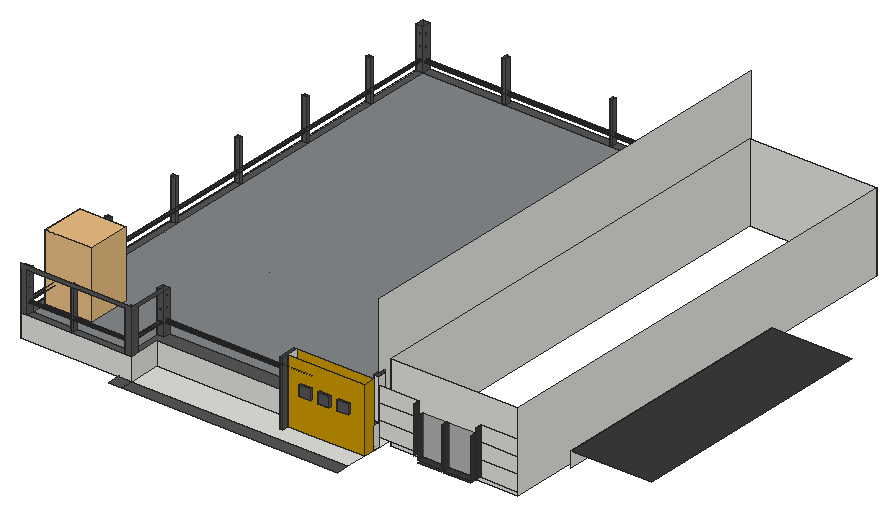
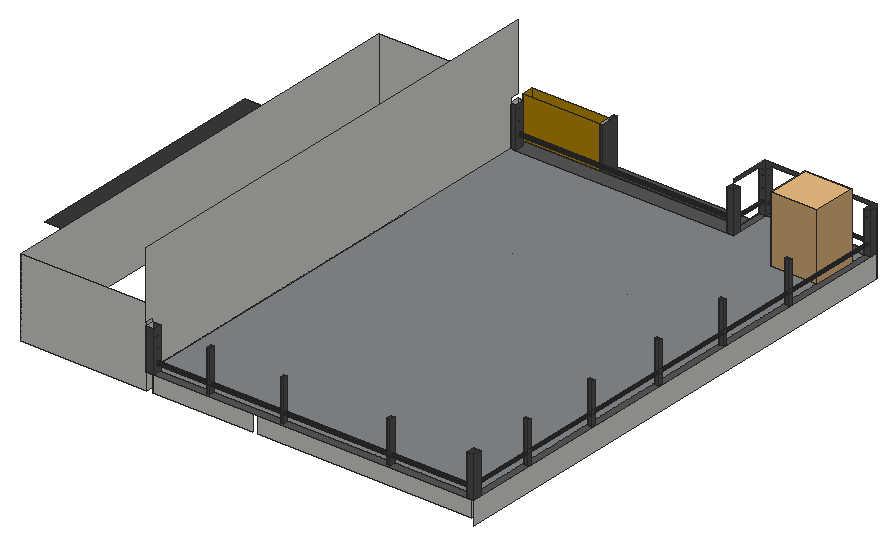
# SketchUp Ruby script. Lengths in inches.
U = 1.inch
M = Sketchup.active_model
def pt(a) = Geom::Point3d.new(a.map { |v| v * U })
def face(e, loops, mat)
  f = e.add_face(loops[0].map { |a| pt(a) })
  loops[1..].each { |l| e.add_face(l.map { |a| pt(a) }).erase! }
  f.material = f.back_material = mat if mat
  f
end
# faces: each face lists its corners as indices into pts; further lists are holes
def faces(e, pts, list, mat = nil) = list.each { |f| face(e, (f[0].is_a?(Array) ? f : [f]).map { |l| l.map { |i| pts[i] } }, mat) }
# xy, xz, yz: faces in a plane at the given z, y or x. An outline is a flat list of corners, or four numbers for a rectangle; further outlines are holes
def ring(l) = l.size == 4 ? [[l[0], l[1]], [l[2], l[1]], [l[2], l[3]], [l[0], l[3]]] : l.each_slice(2).to_a
def flat(e, list, mat, &to3) = list.each { |f| face(e, (f[0].is_a?(Array) ? f : [f]).map { |l| ring(l).map { |u, v| to3.(u, v) } }, mat) }
def xy(e, z, list, mat = nil) = flat(e, list, mat) { |x, y| [x, y, z] }
def xz(e, y, list, mat = nil) = flat(e, list, mat) { |x, z| [x, y, z] }
def yz(e, x, list, mat = nil) = flat(e, list, mat) { |y, z| [x, y, z] }
def lines(e, pts, list) = list.each { |a, b| e.add_line(pt(pts[a]), pt(pts[b])) }
# prism: a flat outline (further loops are holes) pulled along v
def prism(e, loops, v, mat = nil)
  f = face(e, loops, mat); d = Geom::Vector3d.new(v.map { |x| x * U })
  f.pushpull(f.normal.samedirection?(d) ? d.length : -d.length)
end
def box(e, o, s, mat = nil) = prism(e, [[o, [o[0] + s[0], o[1], o[2]], [o[0] + s[0], o[1] + s[1], o[2]], [o[0], o[1] + s[1], o[2]]]], [0, 0, s[2]], mat)
def at(x, y, z, deg = 0) = Geom::Transformation.translation(pt([x, y, z])) * Geom::Transformation.rotation(ORIGIN, Z_AXIS, deg.degrees)
def axes(o, x, y, z) = Geom::Transformation.new([*x, 0, *y, 0, *z, 0, *pt(o).to_a, 1])
def part(name) = M.definitions.add(name)
# library, detail: a bought-in or finely detailed component or shape, given as its bounding box
def library(name, o, s) = part(name).tap { |d| box(d.entities, o, s) }
def detail(e, o, s) = box(e.add_group.entities, o, s)
def put(e, d, t, mat = nil) = e.add_instance(d, t).tap { |i| i.material = mat if mat }
def group(e, t, mat = nil) = e.add_group.tap { |g| g.transformation = t; g.material = mat if mat }.entities
root = M.entities
M.materials.add("[Blacktop Old 01]").color = [132, 136, 139]
M.materials.add("[Color D06]").color = [204, 153, 0]
M.materials.add("[Color M06]").color = [86, 86, 86]
M.materials.add("[Color M07]").color = [58, 58, 58]
M.materials.add("[Translucent Glass Gray]").color = [128, 128, 128]
M.materials["[Translucent Glass Gray]"].alpha = 0.5
c1 = library("Palmera",[-29.85,-16.35,0],[49.71,46.52,62.87])
xy(root,298,[[120,106.4375,352,106.4375,352,128.03,269.98,128.03,269.98,121.03,266.86,121.03,266.86,140.23,120,140.23],[9,115.4375,114,290.0625],[266.86,121.03,269.98,140.23],[269.98,128.03,352,140.23],[120,140.23,236,290.0625],
  [236,140.23,352,290.0625]])
xy(root,298,[[105.8,92.4375,120,106.4375],[120,92.4375,352,106.4375]],"[Color M06]")
xy(root,302.9,[[399.25,141.23,424.3125,147.79],[427.08,141.23,456,147.79]],"[Color M07]")
xy(root,304.98,[[399.25,141.23,424.3125,147.79],[427.08,141.23,456,147.79]],"[Color M07]")
xy(root,315,[[500,220.28,586.5,489.49]],"[Color M07]")
xy(root,318,[[9,296.0625,238.75,637.4375],[244.75,296.0625,352,637.4375]])
xy(root,322,[[0,106.4375,7.24,113.71],[112.36,106.4375,120,113.71],[346.24,147.79,352,156.79],[1.32,218.77,6.25,221.71],[1.32,307.08,6.25,310.02],
  [1.32,393.08,6.25,396.02],[1.32,483.08,6.25,486.02],[1.32,568.77,6.25,571.71],[0,637.4375,7.24,646.4375],[343.33,637.4375,352,646.4375],
  [92.17,637.86,95.73,643.55],[206.23,639.05,209.79,643.61]])
xy(root,322,[[7.24,113.71,112.36,113.71,112.36,156.79,352,156.79,352,637.4375,7.24,637.4375]],"[Blacktop Old 01]")
xy(root,322,[[[7.24,106.4375,112.36,113.71],[52.52,108.5,56.02,112.75]],[[0,113.71,7.24,637.4375],[1.32,218.77,6.25,221.71],[1.32,568.77,6.25,571.71],[1.32,483.08,6.25,486.02],[1.32,393.08,6.25,396.02],[1.32,307.08,6.25,310.02]],[112.36,113.71,120,113.71,120,140.23,352,140.23,352,147.79,346.24,147.79,346.24,156.79,120,156.79,120,149.1,112.36,149.1],[[7.24,637.4375,343.33,646.4375],[285.6,637.86,289.17,643.61],[92.17,637.86,95.73,643.55],[206.23,639.05,209.79,643.61]]],"[Color M06]")
xy(root,333,[[283.87,125.84,295.81,128.03],[304,125.84,315.93,128.03],[324.62,125.84,336.56,128.03]],"[Color M06]")
xy(root,334.51,[[3.85,113.71,4.24,637.4375]],"[Color M06]")
xz(root,106.4375,[[0,298,120,322]])
xz(root,106.4375,[[0,322,7.24,322,7.24,366.125,112.36,366.125,112.36,322,120,322,120,370,0,370]],"[Color M06]")
xz(root,108.5,[[52.52,322,56.02,366.125]],"[Color M06]")
xz(root,112.75,[[52.52,322,56.02,366.125]],"[Color M06]")
xz(root,113.71,[[116.05,333.29,116.46,333.3125,116.84,333.4375,117.1875,333.66,117.46,333.96,117.65,334.33,117.73,334.73,117.71,335.13,117.58,335.52,117.36,335.86,117.06,336.14,116.69,336.32,116.3,336.41,115.89,336.39,115.5,336.26,115.16,336.04,114.89,335.73,114.7,335.37,114.62,334.97,114.64,334.56,114.76,334.18,114.98,333.83,115.29,333.5625,115.65,333.375]])
xz(root,113.71,[[[0,322,7.24,366.125],[4.17,331.53,4.55,331.625,4.9,331.8125,5.18,332.08,5.38,332.42,5.49,332.79,5.5,333.19,5.41,333.57,5.22,333.91,4.95,334.19,4.61,334.4,4.24,334.51,3.85,334.51,3.47,334.42,3.125,334.23,2.84,333.96,2.64,333.63,2.53,333.25,2.52,332.86,2.61,332.48,2.8,332.14,3.07,331.85,3.4,331.65,3.78,331.54],[4.17,357.09,4.55,357.1875,4.9,357.375,5.18,357.65,5.38,357.98,5.49,358.36,5.5,358.75,5.41,359.13,5.22,359.47,4.95,359.75,4.61,359.96,4.24,360.07,3.85,360.08,3.47,359.98,3.125,359.8,2.84,359.53,2.64,359.19,2.53,358.82,2.52,358.42,2.61,358.04,2.8,357.7,3.07,357.42,3.4,357.21,3.78,357.1]],[[112.36,322,120,366.125],[116.05,358.29,116.46,358.3125,116.84,358.4375,117.1875,358.66,117.46,358.96,117.65,359.33,117.73,359.73,117.71,360.13,117.58,360.52,117.36,360.86,117.06,361.14,116.69,361.32,116.3,361.41,115.89,361.39,115.5,361.26,115.16,361.04,114.89,360.73,114.7,360.37,114.62,359.97,114.64,359.56,114.76,359.18,114.98,358.83,115.29,358.5625,115.65,358.375],[116.05,345.98,116.46,346,116.84,346.125,117.1875,346.35,117.46,346.65,117.65,347.01,117.73,347.41,117.71,347.82,117.58,348.21,117.36,348.55,117.06,348.82,116.69,349.01,116.3,349.09,115.89,349.07,115.5,348.95,115.16,348.72,114.89,348.42,114.7,348.06,114.62,347.66,114.64,347.25,114.76,346.86,114.98,346.52,115.29,346.25,115.65,346.0625],[116.05,333.29,116.46,333.3125,116.84,333.4375,117.1875,333.66,117.46,333.96,117.65,334.33,117.73,334.73,117.71,335.13,117.58,335.52,117.36,335.86,117.06,336.14,116.69,336.32,116.3,336.41,115.89,336.39,115.5,336.26,115.16,336.04,114.89,335.73,114.7,335.37,114.62,334.97,114.64,334.56,114.76,334.18,114.98,333.83,115.29,333.5625,115.65,333.375]]],"[Color M06]")
xz(root,121.03,[[266.86,298,269.98,367.0625]],"[Color M06]")
xz(root,125.84,[[283.87,333,295.81,343.87],[304,333,315.93,343.87],[324.62,333,336.56,343.87]],"[Color M06]")
xz(root,128.03,[[[269.98,298,352,367.0625],[283.87,333,295.81,343.87],[304,333,315.93,343.87],[324.62,333,336.56,343.87]]],"[Color D06]")
xz(root,128.03,[[283.87,333,295.81,343.87],[304,333,315.93,343.87],[324.62,333,336.56,343.87]],"[Color M06]")
xz(root,140.23,[[120,298,266.86,322],[266.86,298,269.98,322],[269.98,298,352,322]])
xz(root,140.23,[[269.98,322,352,367.0625]],"[Color D06]")
xz(root,140.23,[[266.86,322,269.98,367.0625]],"[Color M06]")
xz(root,147.79,[[352,307.6,394.33,324.35],[460.92,307.6,500,324.35],[346.24,322,352,366.125],[352,324.35,394.33,341.1],[460.92,324.35,500,341.1],
  [352,341.1,394.33,357.85],[460.92,341.1,500,357.85]])
xz(root,147.79,[[399.25,304.98,424.3125,348.22],[427.08,304.98,456,348.22]],"[Translucent Glass Gray]")
xz(root,149.1,[[[112.36,322,120,366.125],[116.05,345.98,115.65,346.0625,115.29,346.25,114.98,346.52,114.76,346.86,114.64,347.25,114.62,347.66,114.7,348.06,114.89,348.42,115.16,348.72,115.5,348.95,115.89,349.07,116.3,349.09,116.69,349.01,117.06,348.82,117.36,348.55,117.58,348.21,117.71,347.82,117.73,347.41,117.65,347.01,117.46,346.65,117.1875,346.35,116.84,346.125,116.46,346],[116.05,333.29,115.65,333.375,115.29,333.5625,114.98,333.83,114.76,334.18,114.64,334.56,114.62,334.97,114.7,335.37,114.89,335.73,115.16,336.04,115.5,336.26,115.89,336.39,116.3,336.41,116.69,336.32,117.06,336.14,117.36,335.86,117.58,335.52,117.71,335.13,117.73,334.73,117.65,334.33,117.46,333.96,117.1875,333.66,116.84,333.4375,116.46,333.3125]]],"[Color M06]")
xz(root,155.92,[[358,298,494,382]])
xz(root,156.79,[[112.36,322,120,366.125],[346.24,322,352,366.125]],"[Color M06]")
xz(root,218.77,[[1.32,322,6.25,366.125]],"[Color M06]")
xz(root,221.71,[[1.32,322,6.25,366.125]],"[Color M06]")
xz(root,296.0625,[[9,298,238.75,318],[244.75,298,352,318]])
xz(root,307.08,[[1.32,322,6.25,366.125]],"[Color M06]")
xz(root,310.02,[[1.32,322,6.25,366.125]],"[Color M06]")
xz(root,393.08,[[1.32,322,6.25,366.125]],"[Color M06]")
xz(root,396.02,[[1.32,322,6.25,366.125]],"[Color M06]")
xz(root,483.08,[[1.32,322,6.25,366.125]],"[Color M06]")
xz(root,486.02,[[1.32,322,6.25,366.125]],"[Color M06]")
xz(root,568.77,[[1.32,322,6.25,366.125]],"[Color M06]")
xz(root,571.71,[[1.32,322,6.25,366.125]],"[Color M06]")
xz(root,637.4375,[[9,298,238.75,318],[244.75,298,352,318],[358,298,494,382],[4.17,331.53,3.78,331.54,3.4,331.65,3.07,331.85,2.8,332.14,2.61,332.48,2.52,332.86,2.53,333.25,2.64,333.63,2.84,333.96,3.125,334.23,3.47,334.42,3.85,334.51,4.24,334.51,4.61,334.4,4.95,334.19,5.22,333.91,5.41,333.57,5.5,333.19,5.49,332.79,5.38,332.42,5.18,332.08,4.9,331.8125,4.55,331.625]])
xz(root,637.4375,[[[0,322,7.24,366.125],[4.17,357.09,3.78,357.1,3.4,357.21,3.07,357.42,2.8,357.7,2.61,358.04,2.52,358.42,2.53,358.82,2.64,359.19,2.84,359.53,3.125,359.8,3.47,359.98,3.85,360.08,4.24,360.07,4.61,359.96,4.95,359.75,5.22,359.47,5.41,359.13,5.5,358.75,5.49,358.36,5.38,357.98,5.18,357.65,4.9,357.375,4.55,357.1875],[4.17,344.78,3.78,344.79,3.4,344.9,3.07,345.1,2.8,345.39,2.61,345.73,2.52,346.11,2.53,346.5,2.64,346.88,2.84,347.21,3.125,347.48,3.47,347.67,3.85,347.76,4.24,347.76,4.61,347.65,4.95,347.44,5.22,347.16,5.41,346.82,5.5,346.44,5.49,346.04,5.38,345.67,5.18,345.33,4.9,345.0625,4.55,344.875],[4.17,331.53,3.78,331.54,3.4,331.65,3.07,331.85,2.8,332.14,2.61,332.48,2.52,332.86,2.53,333.25,2.64,333.63,2.84,333.96,3.125,334.23,3.47,334.42,3.85,334.51,4.24,334.51,4.61,334.4,4.95,334.19,5.22,333.91,5.41,333.57,5.5,333.19,5.49,332.79,5.38,332.42,5.18,332.08,4.9,331.8125,4.55,331.625]],[343.33,322,352,366.125]],"[Color M06]")
xz(root,637.86,[[92.17,322,95.73,366.125],[285.6,322,289.17,366.125]],"[Color M06]")
xz(root,639.05,[[206.23,322,209.79,366]],"[Color M06]")
xz(root,643.55,[[92.17,322,95.73,366.125]],"[Color M06]")
xz(root,643.61,[[206.23,322,209.79,366],[285.6,322,289.17,366.125]],"[Color M06]")
xz(root,646.4375,[[0,322,7.24,366.125],[343.33,322,352,366.125]],"[Color M06]")
yz(root,0,[[106.4375,298,646.4375,322]])
yz(root,0,[[106.4375,322,113.71,366.125],[637.4375,322,646.4375,366.125]],"[Color M06]")
yz(root,1.32,[[218.77,322,221.71,366.125],[307.08,322,310.02,366.125],[393.08,322,396.02,366.125],[483.08,322,486.02,366.125],[568.77,322,571.71,366.125]],"[Color M06]")
yz(root,6.25,[[218.77,322,221.71,366.125],[307.08,322,310.02,366.125],[393.08,322,396.02,366.125],[483.08,322,486.02,366.125],[568.77,322,571.71,366.125]],"[Color M06]")
yz(root,7.08,[[641.59,329.73,641.125,329.79,640.6875,329.97,640.3125,330.26,640.03,330.63,639.84,331.07,639.78,331.54,639.84,332.01,640.03,332.45,640.3125,332.82,640.6875,333.11,641.125,333.29,641.59,333.35,642.0625,333.29,642.5,333.11,642.875,332.82,643.16,332.45,643.35,332.01,643.41,331.54,643.35,331.07,643.16,330.63,642.875,330.26,642.5,329.97,642.0625,329.79]])
yz(root,7.24,[[110.32,332.4,109.9375,332.45,109.57,332.6,109.26,332.84,109.03,333.15,108.875,333.51,108.82,333.9,108.875,334.28,109.03,334.65,109.26,334.96,109.57,335.19,109.9375,335.34,110.32,335.4,110.71,335.34,111.07,335.19,111.38,334.96,111.625,334.65,111.77,334.28,111.82,333.9,111.77,333.51,111.625,333.15,111.38,332.84,111.07,332.6,110.71,332.45]])
yz(root,7.24,[[[106.4375,322,113.71,366.125],[110.32,357.9,109.9375,357.95,109.57,358.1,109.26,358.34,109.03,358.65,108.875,359.01,108.82,359.4,108.875,359.78,109.03,360.15,109.26,360.46,109.57,360.69,109.9375,360.84,110.32,360.9,110.71,360.84,111.07,360.69,111.38,360.46,111.625,360.15,111.77,359.78,111.82,359.4,111.77,359.01,111.625,358.65,111.38,358.34,111.07,358.1,110.71,357.95],[110.32,345.27,109.9375,345.32,109.57,345.47,109.26,345.71,109.03,346.02,108.875,346.38,108.82,346.77,108.875,347.16,109.03,347.52,109.26,347.83,109.57,348.07,109.9375,348.22,110.32,348.27,110.71,348.22,111.07,348.07,111.38,347.83,111.625,347.52,111.77,347.16,111.82,346.77,111.77,346.38,111.625,346.02,111.38,345.71,111.07,345.47,110.71,345.32],[110.32,332.4,109.9375,332.45,109.57,332.6,109.26,332.84,109.03,333.15,108.875,333.51,108.82,333.9,108.875,334.28,109.03,334.65,109.26,334.96,109.57,335.19,109.9375,335.34,110.32,335.4,110.71,335.34,111.07,335.19,111.38,334.96,111.625,334.65,111.77,334.28,111.82,333.9,111.77,333.51,111.625,333.15,111.38,332.84,111.07,332.6,110.71,332.45]],[[637.4375,322,646.4375,366.125],[641.59,343.41,641.125,343.48,640.6875,343.66,640.3125,343.94,640.03,344.32,639.84,344.76,639.78,345.23,639.84,345.7,640.03,346.13,640.3125,346.51,640.6875,346.8,641.125,346.98,641.59,347.04,642.0625,346.98,642.5,346.8,642.875,346.51,643.16,346.13,643.35,345.7,643.41,345.23,643.35,344.76,643.16,344.32,642.875,343.94,642.5,343.66,642.0625,343.48],[641.59,355.85,641.125,355.91,640.6875,356.09,640.3125,356.38,640.03,356.76,639.84,357.19,639.78,357.66,639.84,358.13,640.03,358.57,640.3125,358.95,640.6875,359.23,641.125,359.41,641.59,359.48,642.0625,359.41,642.5,359.23,642.875,358.95,643.16,358.57,643.35,358.13,643.41,357.66,643.35,357.19,643.16,356.76,642.875,356.38,642.5,356.09,642.0625,355.91]]],"[Color M06]")
yz(root,9,[[296.0625,298,637.4375,318]])
yz(root,52.52,[[108.5,322,112.75,366.125]],"[Color M06]")
yz(root,56.02,[[108.5,322,112.75,366.125]],"[Color M06]")
yz(root,92.17,[[637.86,322,643.55,366.125]],"[Color M06]")
yz(root,95.73,[[637.86,322,643.55,366.125]],"[Color M06]")
yz(root,112.36,[[[106.4375,322,113.71,366.125],[110.32,357.9,110.71,357.95,111.07,358.1,111.38,358.34,111.625,358.65,111.77,359.01,111.82,359.4,111.77,359.78,111.625,360.15,111.38,360.46,111.07,360.69,110.71,360.84,110.32,360.9,109.9375,360.84,109.57,360.69,109.26,360.46,109.03,360.15,108.875,359.78,108.82,359.4,108.875,359.01,109.03,358.65,109.26,358.34,109.57,358.1,109.9375,357.95]],[149.1,322,156.79,366.125]],"[Color M06]")
yz(root,112.49,[[110.32,332.4,110.71,332.45,111.07,332.6,111.38,332.84,111.625,333.15,111.77,333.51,111.82,333.9,111.77,334.28,111.625,334.65,111.38,334.96,111.07,335.19,110.71,335.34,110.32,335.4,109.9375,335.34,109.57,335.19,109.26,334.96,109.03,334.65,108.875,334.28,108.82,333.9,108.875,333.51,109.03,333.15,109.26,332.84,109.57,332.6,109.9375,332.45]])
yz(root,120,[[106.4375,298,140.23,322],[152.72,334.31,152.32,334.36,151.94,334.52,151.62,334.77,151.37,335.09,151.21,335.47,151.16,335.87,151.21,336.28,151.37,336.65,151.62,336.98,151.94,337.22,152.32,337.38,152.72,337.43,153.125,337.38,153.5,337.22,153.83,336.98,154.07,336.65,154.23,336.28,154.28,335.87,154.23,335.47,154.07,335.09,153.83,334.77,153.5,334.52,153.125,334.36]])
yz(root,120,[[106.4375,322,113.71,322,113.71,366.125,147.79,366.125,147.79,370,106.4375,370],[[149.1,322,156.79,366.125],[152.72,358.93,152.32,358.99,151.94,359.14,151.62,359.39,151.37,359.71,151.21,360.09,151.16,360.5,151.21,360.9,151.37,361.28,151.62,361.6,151.94,361.85,152.32,362,152.72,362.06,153.125,362,153.5,361.85,153.83,361.6,154.07,361.28,154.23,360.9,154.28,360.5,154.23,360.09,154.07,359.71,153.83,359.39,153.5,359.14,153.125,358.99],[152.72,347.12,152.32,347.17,151.94,347.33,151.62,347.58,151.37,347.9,151.21,348.28,151.16,348.68,151.21,349.09,151.37,349.46,151.62,349.79,151.94,350.04,152.32,350.19,152.72,350.25,153.125,350.19,153.5,350.04,153.83,349.79,154.07,349.46,154.23,349.09,154.28,348.68,154.23,348.28,154.07,347.9,153.83,347.58,153.5,347.33,153.125,347.17],[152.72,334.31,152.32,334.36,151.94,334.52,151.62,334.77,151.37,335.09,151.21,335.47,151.16,335.87,151.21,336.28,151.37,336.65,151.62,336.98,151.94,337.22,152.32,337.38,152.72,337.43,153.125,337.38,153.5,337.22,153.83,336.98,154.07,336.65,154.23,336.28,154.28,335.87,154.23,335.47,154.07,335.09,153.83,334.77,153.5,334.52,153.125,334.36]]],"[Color M06]")
yz(root,206.23,[[639.05,322,643.61,366]],"[Color M06]")
yz(root,209.79,[[639.05,322,643.61,366]],"[Color M06]")
yz(root,266.86,[[121.03,298,140.23,367.0625]],"[Color M06]")
yz(root,269.98,[[128.03,298,140.23,367.0625]])
yz(root,269.98,[[121.03,298,128.03,367.0625]],"[Color M06]")
yz(root,283.87,[[125.84,333,128.03,343.87]],"[Color M06]")
yz(root,285.6,[[637.86,322,643.61,366.125]],"[Color M06]")
yz(root,289.17,[[637.86,322,643.61,366.125]],"[Color M06]")
yz(root,295.81,[[125.84,333,128.03,343.87]],"[Color M06]")
yz(root,304,[[125.84,333,128.03,343.87]],"[Color M06]")
yz(root,315.93,[[125.84,333,128.03,343.87]],"[Color M06]")
yz(root,324.62,[[125.84,333,128.03,343.87]],"[Color M06]")
yz(root,336.56,[[125.84,333,128.03,343.87]],"[Color M06]")
yz(root,343.33,[[641.59,329.73,642.0625,329.79,642.5,329.97,642.875,330.26,643.16,330.63,643.35,331.07,643.41,331.54,643.35,332.01,643.16,332.45,642.875,332.82,642.5,333.11,642.0625,333.29,641.59,333.35,641.125,333.29,640.6875,333.11,640.3125,332.82,640.03,332.45,639.84,332.01,639.78,331.54,639.84,331.07,640.03,330.63,640.3125,330.26,640.6875,329.97,641.125,329.79]])
yz(root,343.33,[[[637.4375,322,646.4375,366.125],[641.59,355.85,642.0625,355.91,642.5,356.09,642.875,356.38,643.16,356.76,643.35,357.19,643.41,357.66,643.35,358.13,643.16,358.57,642.875,358.95,642.5,359.23,642.0625,359.41,641.59,359.48,641.125,359.41,640.6875,359.23,640.3125,358.95,640.03,358.57,639.84,358.13,639.78,357.66,639.84,357.19,640.03,356.76,640.3125,356.38,640.6875,356.09,641.125,355.91],[641.59,343.41,642.0625,343.48,642.5,343.66,642.875,343.94,643.16,344.32,643.35,344.76,643.41,345.23,643.35,345.7,643.16,346.13,642.875,346.51,642.5,346.8,642.0625,346.98,641.59,347.04,641.125,346.98,640.6875,346.8,640.3125,346.51,640.03,346.13,639.84,345.7,639.78,345.23,639.84,344.76,640.03,344.32,640.3125,343.94,640.6875,343.66,641.125,343.48],[641.59,329.73,642.0625,329.79,642.5,329.97,642.875,330.26,643.16,330.63,643.35,331.07,643.41,331.54,643.35,332.01,643.16,332.45,642.875,332.82,642.5,333.11,642.0625,333.29,641.59,333.35,641.125,333.29,640.6875,333.11,640.3125,332.82,640.03,332.45,639.84,332.01,639.78,331.54,639.84,331.07,640.03,330.63,640.3125,330.26,640.6875,329.97,641.125,329.79]]],"[Color M06]")
yz(root,346.24,[[[147.79,322,156.79,366.125],[152.72,347.12,153.125,347.17,153.5,347.33,153.83,347.58,154.07,347.9,154.23,348.28,154.28,348.68,154.23,349.09,154.07,349.46,153.83,349.79,153.5,350.04,153.125,350.19,152.72,350.25,152.32,350.19,151.94,350.04,151.62,349.79,151.37,349.46,151.21,349.09,151.16,348.68,151.21,348.28,151.37,347.9,151.62,347.58,151.94,347.33,152.32,347.17],[152.72,358.93,153.125,358.99,153.5,359.14,153.83,359.39,154.07,359.71,154.23,360.09,154.28,360.5,154.23,360.9,154.07,361.28,153.83,361.6,153.5,361.85,153.125,362,152.72,362.06,152.32,362,151.94,361.85,151.62,361.6,151.37,361.28,151.21,360.9,151.16,360.5,151.21,360.09,151.37,359.71,151.62,359.39,151.94,359.14,152.32,358.99]]],"[Color M06]")
yz(root,346.3125,[[152.72,334.31,153.125,334.36,153.5,334.52,153.83,334.77,154.07,335.09,154.23,335.47,154.28,335.87,154.23,336.28,154.07,336.65,153.83,336.98,153.5,337.22,153.125,337.38,152.72,337.43,152.32,337.38,151.94,337.22,151.62,336.98,151.37,336.65,151.21,336.28,151.16,335.87,151.21,335.47,151.37,335.09,151.62,334.77,151.94,334.52,152.32,334.36]])
yz(root,352,[[140.23,298,147.79,322],[296.0625,298,637.4375,318],[296.0625,318,637.4375,322],[147.79,322,156.79,366.125],[156.79,322,156.79,370,147.79,370,147.79,441.0625,646.4375,441.0625,646.4375,370,637.4375,370,637.4375,322],
  [637.4375,322,646.4375,366.125]])
yz(root,352,[[128.03,298,140.23,367.0625]],"[Color D06]")
yz(root,358,[[155.92,298,637.4375,382]])
yz(root,394.33,[[141.23,307.6,147.79,324.35],[141.23,324.35,147.79,341.1],[141.23,341.1,147.79,357.85]],"[Color M07]")
yz(root,399.25,[[141.23,304.98,147.79,348.22]],"[Color M07]")
yz(root,424.3125,[[141.23,304.98,147.79,348.22]],"[Color M07]")
yz(root,427.08,[[141.23,304.98,147.79,348.22]],"[Color M07]")
yz(root,456,[[141.23,304.98,147.79,348.22]],"[Color M07]")
yz(root,460.92,[[141.23,307.6,147.79,324.35],[141.23,324.35,147.79,341.1],[141.23,341.1,147.79,357.85]],"[Color M07]")
yz(root,494,[[155.92,298,637.4375,382]])
yz(root,500,[[220.28,298,489.49,315]])
p = [[343.33,641.59,329.73],[343.33,641.125,329.79],[7.08,641.125,329.79],[7.08,641.59,329.73],[343.33,642.0625,329.79],[7.08,642.0625,329.79],
  [343.33,640.6875,329.97],[7.08,640.6875,329.97],[343.33,642.5,329.97],[7.08,642.5,329.97],[343.33,640.3125,330.26],[7.08,640.3125,330.26],
  [343.33,642.875,330.26],[7.08,642.875,330.26],[343.33,640.03,330.63],[7.08,640.03,330.63],[343.33,643.16,330.63],[7.08,643.16,330.63],
  [343.33,639.84,331.07],[7.08,639.84,331.07],[343.33,643.35,331.07],[7.08,643.35,331.07],[343.33,639.78,331.54],[7.08,639.78,331.54],
  [343.33,643.41,331.54],[7.08,643.41,331.54],[3.4,637.4375,331.65],[3.78,637.4375,331.54],[3.78,113.71,331.54],[3.4,113.71,331.65],
  [4.17,637.4375,331.53],[4.17,113.71,331.53],[4.55,637.4375,331.625],[4.55,113.71,331.625],[343.33,639.84,332.01],[7.08,639.84,332.01],
  [343.33,643.35,332.01],[7.08,643.35,332.01],[4.9,637.4375,331.8125],[4.9,113.71,331.8125],[3.07,637.4375,331.85],[3.07,113.71,331.85],
  [5.18,637.4375,332.08],[5.18,113.71,332.08],[2.8,637.4375,332.14],[2.8,113.71,332.14],[343.33,640.03,332.45],[7.08,640.03,332.45],
  [343.33,643.16,332.45],[7.08,643.16,332.45],[2.61,637.4375,332.48],[2.61,113.71,332.48],[5.38,637.4375,332.42],[5.38,113.71,332.42],
  [7.24,109.57,332.6],[7.24,109.9375,332.45],[112.49,109.9375,332.45],[112.49,109.57,332.6],[7.24,110.32,332.4],[112.49,110.32,332.4],
  [7.24,110.71,332.45],[112.49,110.71,332.45],[7.24,111.07,332.6],[112.49,111.07,332.6],[5.49,637.4375,332.79],[5.49,113.71,332.79],
  [343.33,640.3125,332.82],[7.08,640.3125,332.82],[343.33,642.875,332.82],[7.08,642.875,332.82],[2.52,637.4375,332.86],[2.52,113.71,332.86],
  [7.24,109.26,332.84],[112.49,109.26,332.84],[7.24,111.38,332.84],[112.49,111.38,332.84],[7.24,109.03,333.15],[112.49,109.03,333.15],
  [7.24,111.625,333.15],[112.49,111.625,333.15],[5.5,637.4375,333.19],[5.5,113.71,333.19],[343.33,640.6875,333.11],[7.08,640.6875,333.11],
  [343.33,642.5,333.11],[7.08,642.5,333.11],[2.53,637.4375,333.25],[2.53,113.71,333.25],[7.24,108.875,333.51],[112.49,108.875,333.51],
  [7.24,111.77,333.51],[112.49,111.77,333.51],[343.33,641.125,333.29],[7.08,641.125,333.29],[343.33,642.0625,333.29],[7.08,642.0625,333.29],
  [5.41,637.4375,333.57],[5.41,113.71,333.57],[2.64,637.4375,333.63],[2.64,113.71,333.63],[116.05,113.71,333.29],[115.65,113.71,333.375],
  [115.65,149.1,333.375],[116.05,149.1,333.29],[116.46,113.71,333.3125],[116.46,149.1,333.3125],[116.84,113.71,333.4375],[116.84,149.1,333.4375],
  [343.33,641.59,333.35],[7.08,641.59,333.35],[115.29,113.71,333.5625],[115.29,149.1,333.5625],[117.1875,113.71,333.66],[117.1875,149.1,333.66],
  [7.24,108.82,333.9],[112.49,108.82,333.9],[7.24,111.82,333.9],[112.49,111.82,333.9],[2.84,637.4375,333.96],[2.84,113.71,333.96],
  [5.22,637.4375,333.91],[5.22,113.71,333.91],[114.98,113.71,333.83],[114.98,149.1,333.83],[117.46,113.71,333.96],[117.46,149.1,333.96],
  [114.76,113.71,334.18],[114.76,149.1,334.18],[7.24,108.875,334.28],[112.49,108.875,334.28],[7.24,111.77,334.28],[112.49,111.77,334.28],
  [4.95,637.4375,334.19],[4.95,113.71,334.19],[3.125,637.4375,334.23],[3.125,113.71,334.23],[117.65,113.71,334.33],[117.65,149.1,334.33],
  [3.47,637.4375,334.42],[3.47,113.71,334.42],[4.61,637.4375,334.4],[4.61,113.71,334.4],[114.64,113.71,334.56],[114.64,149.1,334.56],
  [7.24,109.03,334.65],[112.49,109.03,334.65],[7.24,111.625,334.65],[112.49,111.625,334.65],[117.73,113.71,334.73],[117.73,149.1,334.73],
  [120,152.32,334.36],[120,152.72,334.31],[346.3125,152.72,334.31],[346.3125,152.32,334.36],[120,153.125,334.36],[346.3125,153.125,334.36],
  [3.85,637.4375,334.51],[3.85,113.71,334.51],[4.24,637.4375,334.51],[4.24,113.71,334.51],[120,151.94,334.52],[346.3125,151.94,334.52],
  [120,153.5,334.52],[346.3125,153.5,334.52],[120,151.62,334.77],[346.3125,151.62,334.77],[120,153.83,334.77],[346.3125,153.83,334.77],
  [7.24,109.26,334.96],[112.49,109.26,334.96],[7.24,111.38,334.96],[112.49,111.38,334.96],[114.62,113.71,334.97],[114.62,149.1,334.97],
  [117.71,113.71,335.13],[117.71,149.1,335.13],[120,151.37,335.09],[346.3125,151.37,335.09],[120,154.07,335.09],[346.3125,154.07,335.09],
  [7.24,109.57,335.19],[112.49,109.57,335.19],[7.24,111.07,335.19],[112.49,111.07,335.19],[114.7,113.71,335.37],[114.7,149.1,335.37],
  [117.58,113.71,335.52],[117.58,149.1,335.52],[120,151.21,335.47],[346.3125,151.21,335.47],[120,154.23,335.47],[346.3125,154.23,335.47],
  [7.24,109.9375,335.34],[112.49,109.9375,335.34],[7.24,110.71,335.34],[112.49,110.71,335.34],[7.24,110.32,335.4],[112.49,110.32,335.4],
  [114.89,113.71,335.73],[114.89,149.1,335.73],[117.36,113.71,335.86],[117.36,149.1,335.86],[120,151.16,335.87],[346.3125,151.16,335.87],
  [120,154.28,335.87],[346.3125,154.28,335.87],[115.16,113.71,336.04],[115.16,149.1,336.04],[117.06,113.71,336.14],[117.06,149.1,336.14],
  [120,151.21,336.28],[346.3125,151.21,336.28],[120,154.23,336.28],[346.3125,154.23,336.28],[115.5,113.71,336.26],[115.5,149.1,336.26],
  [116.69,113.71,336.32],[116.69,149.1,336.32],[115.89,113.71,336.39],[115.89,149.1,336.39],[116.3,113.71,336.41],[116.3,149.1,336.41],
  [120,151.37,336.65],[346.3125,151.37,336.65],[120,154.07,336.65],[346.3125,154.07,336.65],[120,151.62,336.98],[346.3125,151.62,336.98],
  [120,153.83,336.98],[346.3125,153.83,336.98],[120,151.94,337.22],[346.3125,151.94,337.22],[120,153.5,337.22],[346.3125,153.5,337.22],
  [120,152.32,337.38],[346.3125,152.32,337.38],[120,153.125,337.38],[346.3125,153.125,337.38],[120,152.72,337.43],[346.3125,152.72,337.43],
  [238.75,296.0625,322],[236,290.0625,298],[114,115.4375,298],[114,115.4375,322],[9,115.4375,298],[9,115.4375,322],
  [9,290.0625,298],[9,290.0625,322],[120,290.0625,298],[120,290.0625,322],[43.375,637.4375,322],[43.375,637.4375,318],
  [238.75,637.4375,318],[238.75,637.4375,322],[9,637.4375,318],[9,637.4375,322],[238.75,296.0625,318],[273.5625,637.4375,322],
  [273.5625,637.4375,318]]
faces(root,p,[[0,1,2,3],[4,0,3,5],[1,6,7,2],[8,4,5,9],[6,10,11,7],[12,8,9,13],[10,14,15,11],[16,12,13,17],
  [14,18,19,15],[20,16,17,21],[18,22,23,19],[24,20,21,25],[26,27,28,29],[27,30,31,28],[30,32,33,31],[22,34,35,23],
  [36,24,25,37],[32,38,39,33],[40,26,29,41],[38,42,43,39],[44,40,41,45],[34,46,47,35],[48,36,37,49],[50,44,45,51],
  [42,52,53,43],[54,55,56,57],[55,58,59,56],[58,60,61,59],[60,62,63,61],[52,64,65,53],[46,66,67,47],[68,48,49,69],
  [70,50,51,71],[72,54,57,73],[62,74,75,63],[76,72,73,77],[74,78,79,75],[64,80,81,65],[66,82,83,67],[84,68,69,85],
  [86,70,71,87],[88,76,77,89],[78,90,91,79],[82,92,93,83],[94,84,85,95],[80,96,97,81],[98,86,87,99],[100,101,102,103],
  [104,100,103,105],[106,104,105,107],[92,108,109,93],[108,94,95,109],[101,110,111,102],[112,106,107,113],[114,88,89,115],[90,116,117,91],
  [118,98,99,119],[96,120,121,97],[110,122,123,111],[124,112,113,125],[122,126,127,123],[128,114,115,129],[116,130,131,117],[120,132,133,121],
  [134,118,119,135],[136,124,125,137],[138,134,135,139],[132,140,141,133],[126,142,143,127],[144,128,129,145],[130,146,147,131],[148,136,137,149],
  [150,151,152,153],[151,154,155,152],[156,138,139,157],[140,158,159,141],[160,150,153,161],[154,162,163,155],[164,160,161,165],[162,166,167,163],
  [168,144,145,169],[146,170,171,147],[142,172,173,143],[174,148,149,175],[176,164,165,177],[166,178,179,167],[180,168,169,181],[170,182,183,171],
  [172,184,185,173],[186,174,175,187],[188,176,177,189],[178,190,191,179],[192,180,181,193],[182,194,195,183],[196,192,193,197],[194,196,197,195],
  [184,198,199,185],[200,186,187,201],[202,188,189,203],[190,204,205,191],[198,206,207,199],[208,200,201,209],[210,202,203,211],[204,212,213,205],
  [206,214,215,207],[216,208,209,217],[214,218,219,215],[220,216,217,221],[222,210,211,223],[212,224,225,213],[218,220,221,219],[226,222,223,227],
  [224,228,229,225],[230,226,227,231],[228,232,233,229],[234,230,231,235],[232,236,237,233],[238,234,235,239],[236,238,239,237]],"[Color M06]")
lines(root,p,[[240,241],[242,243],[244,245],[246,247],[248,249],[250,251],[252,253],[254,255],[256,240],[257,258]])
put(root,c1,axes([36.39,147.9,322],[1,0,0],[0,1,0],[0,0,1.13]))
